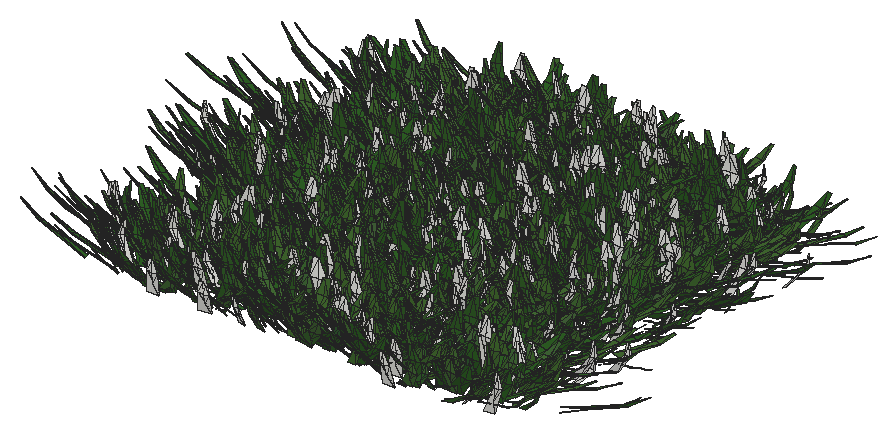
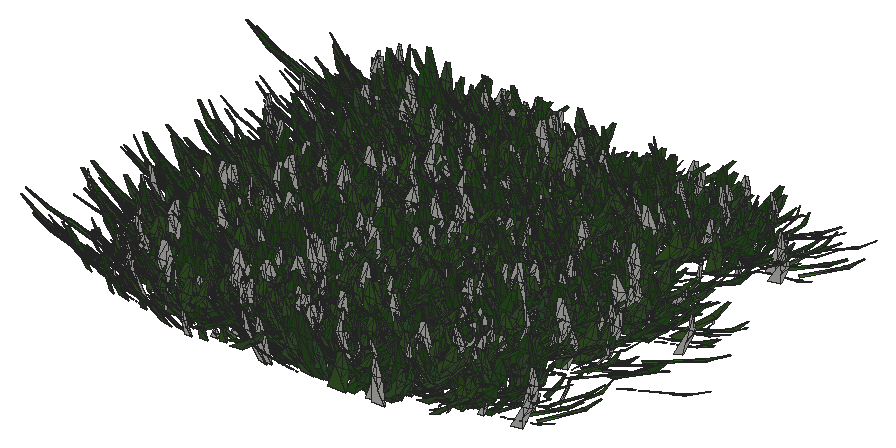
# SketchUp Ruby script. Lengths in inches.
U = 1.inch
M = Sketchup.active_model
def pt(a) = Geom::Point3d.new(a.map { |v| v * U })
def face(e, loops, mat)
  f = e.add_face(loops[0].map { |a| pt(a) })
  loops[1..].each { |l| e.add_face(l.map { |a| pt(a) }).erase! }
  f.material = f.back_material = mat if mat
  f
end
# faces: each face lists its corners as indices into pts; further lists are holes
def faces(e, pts, list, mat = nil) = list.each { |f| face(e, (f[0].is_a?(Array) ? f : [f]).map { |l| l.map { |i| pts[i] } }, mat) }
# xy, xz, yz: faces in a plane at the given z, y or x. An outline is a flat list of corners, or four numbers for a rectangle; further outlines are holes
def ring(l) = l.size == 4 ? [[l[0], l[1]], [l[2], l[1]], [l[2], l[3]], [l[0], l[3]]] : l.each_slice(2).to_a
def flat(e, list, mat, &to3) = list.each { |f| face(e, (f[0].is_a?(Array) ? f : [f]).map { |l| ring(l).map { |u, v| to3.(u, v) } }, mat) }
def xy(e, z, list, mat = nil) = flat(e, list, mat) { |x, y| [x, y, z] }
def xz(e, y, list, mat = nil) = flat(e, list, mat) { |x, z| [x, y, z] }
def yz(e, x, list, mat = nil) = flat(e, list, mat) { |y, z| [x, y, z] }
def lines(e, pts, list) = list.each { |a, b| e.add_line(pt(pts[a]), pt(pts[b])) }
# prism: a flat outline (further loops are holes) pulled along v
def prism(e, loops, v, mat = nil)
  f = face(e, loops, mat); d = Geom::Vector3d.new(v.map { |x| x * U })
  f.pushpull(f.normal.samedirection?(d) ? d.length : -d.length)
end
def box(e, o, s, mat = nil) = prism(e, [[o, [o[0] + s[0], o[1], o[2]], [o[0] + s[0], o[1] + s[1], o[2]], [o[0], o[1] + s[1], o[2]]]], [0, 0, s[2]], mat)
def at(x, y, z, deg = 0) = Geom::Transformation.translation(pt([x, y, z])) * Geom::Transformation.rotation(ORIGIN, Z_AXIS, deg.degrees)
def axes(o, x, y, z) = Geom::Transformation.new([*x, 0, *y, 0, *z, 0, *pt(o).to_a, 1])
def part(name) = M.definitions.add(name)
# library, detail: a bought-in or finely detailed component or shape, given as its bounding box
def library(name, o, s) = part(name).tap { |d| box(d.entities, o, s) }
def detail(e, o, s) = box(e.add_group.entities, o, s)
def put(e, d, t, mat = nil) = e.add_instance(d, t).tap { |i| i.material = mat if mat }
def group(e, t, mat = nil) = e.add_group.tap { |g| g.transformation = t; g.material = mat if mat }.entities
root = M.entities
M.materials.add("Material10").color = [48, 100, 38]
M.materials.add("Material3").color = [68, 110, 58]
M.materials.add("Material4").color = [48, 90, 38]
M.materials.add("Material5").color = [68, 110, 48]
M.materials.add("Material6").color = [48, 90, 48]
M.materials.add("Material7").color = [58, 110, 58]
M.materials.add("Material8").color = [58, 90, 38]
M.materials.add("Material9").color = [68, 100, 58]
c1 = part("grass00")
p = [[-0.6875,0.15,0],[-0.56,0.08,5.52],[-0.04,0.03,2.76],[0.48,-0.02,0],[0.35,-0.02,5.52],[-0.1,-0.14,5.52],
  [-0.12,0.65,8.37],[-0.42,0.65,8.37]]
faces(c1.entities,p,[[0,1,2,3],[3,2,4],[1,5,2],[5,4,2],[1,6,5],[4,5,6],[7,6,1]])
c2 = part("Group16\#1")
put(c2.entities,c1,axes([1.44,-0.61,-0.01],[0.05352,0.12609,0],[-0.10704,0.04543,0.07239],[0.06664,-0.02828,0.11628]),"Material6")
put(c2.entities,c1,axes([0.76,-0.15,-0.01],[0.04676,0.24062,0],[-0.23162,0.04501,0.06642],[0.0652,-0.01267,0.23595]),"Material3")
put(c2.entities,c1,axes([0.79,0.01,-0.01],[-0.00606,0.34651,0],[-0.34381,-0.00602,0.0432],[0.04319,0.00076,0.34386]))
put(c2.entities,c1,axes([1,0.23,-0.01],[-0.07192,0.31144,0],[-0.28722,-0.06632,0.1236],[0.12043,0.02781,0.29478]),"Material5")
put(c2.entities,c1,axes([1.66,0.77,-0.01],[-0.13828,0.29651,0],[-0.21551,-0.1005,0.22471],[0.20365,0.09498,0.23779]),"Material10")
put(c2.entities,c1,axes([0.6875,0.52,-0.01],[-0.18126,0.24051,0],[-0.22746,-0.17142,0.09788],[0.07817,0.05891,0.28481]),"Material5")
put(c2.entities,c1,axes([0.68,0.78,-0.01],[-0.215,0.18688,0],[-0.12385,-0.14248,0.21334],[0.13995,0.16101,0.18878]),"Material3")
put(c2.entities,c1,axes([0.56,1,-0.01],[-0.13756,0.07624,0],[-0.06159,-0.11112,0.0927],[0.04494,0.08108,0.12705]),"Material5")
put(c2.entities,c1,axes([0.2,0.64,-0.01],[-0.23729,0.07254,0],[-0.05711,-0.18681,0.153],[0.04473,0.14632,0.19535]),"Material10")
put(c2.entities,c1,axes([0.0625,0.72,-0.01],[-0.28874,0.02525,0],[-0.02179,-0.24916,0.14647],[0.01276,0.14591,0.25012]),"Material3")
put(c2.entities,c1,axes([-0.08,0.62,-0.01],[-0.34089,-0.04187,0],[0.03255,-0.26504,0.216],[-0.02633,0.21439,0.26703]),"Material10")
put(c2.entities,c1,axes([-0.34,0.98,-0.01],[-0.14314,-0.0493,0],[0.04397,-0.12769,0.06843],[-0.02228,0.0647,0.13505]),"Material10")
put(c2.entities,c1,axes([-0.87,1.45,-0.01],[-0.23488,-0.14114,0],[0.13761,-0.22901,0.06087],[-0.03135,0.05217,0.26717]))
put(c2.entities,c1,axes([-0.72,0.77,-0.01],[-0.14208,-0.13251,0],[0.07209,-0.0773,0.16301],[-0.11118,0.11922,0.1057]),"Material10")
put(c2.entities,c1,axes([-0.62,0.43,-0.01],[-0.14845,-0.21203,0],[0.18654,-0.13061,0.12304],[-0.10079,0.07057,0.22772]),"Material3")
put(c2.entities,c1,axes([-0.68,0.29,-0.01],[-0.13639,-0.32136,0],[0.31723,-0.13464,0.05579],[-0.05136,0.0218,0.34462]),"Material4")
put(c2.entities,c1,axes([-0.64,0.125,-0.01],[-0.0458,-0.23569,0],[0.22124,-0.043,0.08276],[-0.08124,0.01579,0.22538]),"Material7")
put(c2.entities,c1,axes([-1.6,-0.03,-0.01],[0.00576,-0.32897,0],[0.27526,0.00482,0.18018],[-0.18015,-0.00315,0.2753]),"Material5")
put(c2.entities,c1,axes([-1.36,-0.31,-0.01],[0.05718,-0.24765,0],[0.18172,0.04196,0.17267],[-0.16825,-0.03885,0.1865]),"Material10")
put(c2.entities,c1,axes([-1.54,-0.72,-0.01],[0.06537,-0.14017,0],[0.13555,0.06321,0.03939],[-0.0357,-0.01665,0.14956]))
put(c2.entities,c1,axes([-1.19,-0.9,-0.01],[0.09597,-0.12735,0],[0.11214,0.08451,0.07557],[-0.06035,-0.04548,0.14042]),"Material9")
put(c2.entities,c1,axes([-0.47,-0.54,-0.01],[0.11588,-0.10072,0],[0.0618,0.0711,0.12124],[-0.07953,-0.0915,0.0942]))
put(c2.entities,c1,axes([-0.47,-0.84,-0.01],[0.11927,-0.0661,0],[0.06603,0.11913,0.00646],[-0.00313,-0.00565,0.13621]),"Material5")
put(c2.entities,c1,axes([-0.38,-1.24,-0.01],[0.28037,-0.08571,0],[0.0618,0.20215,0.20315],[-0.05939,-0.19428,0.21139]),"Material9")
put(c2.entities,c1,axes([-0.06,-0.66,-0.01],[0.22719,-0.01987,0],[0.01247,0.14255,0.17758],[-0.01547,-0.17691,0.1431]),"Material8")
put(c2.entities,c1,axes([0.11,-0.89,-0.01],[0.14882,0.01828,0],[-0.01058,0.08611,0.12229],[0.01491,-0.12138,0.08676]),"Material6")
put(c2.entities,c1,axes([0.25,-0.72,-0.01],[0.20481,0.07053,0],[-0.06206,0.18022,0.10291],[0.03351,-0.0973,0.1906]),"Material6")
put(c2.entities,c1,axes([0.85,-1.42,-0.01],[0.16481,0.09904,0],[-0.09472,0.15762,0.05616],[0.02893,-0.04814,0.18389]),"Material5")
put(c2.entities,c1,axes([1.01,-1.09,-0.01],[0.21858,0.20385,0],[-0.17495,0.1876,0.15339],[0.10462,-0.11218,0.25652]),"Material10")
put(c2.entities,c1,axes([1.01,-0.71,-0.01],[0.08733,0.12473,0],[-0.06445,0.04512,0.13037],[0.1068,-0.07477,0.07867]),"Material6")
c3 = part("Group15\#1")
put(c3.entities,c2,at(0,0,0))
c4 = part("3darcstudiotree_grass00\#1")
put(c4.entities,c3,at(0,0,0))
put(root,c4,axes([225.51,46.77,7.6],[3.32161,0.35112,0],[-1.50903,0.89222,-0.04149],[-0.12715,0.07518,1.90578]))
put(root,c4,axes([225.43,47.55,7.6],[4.42522,0.39878,0],[-1.59159,1.10387,-0.05978],[-0.10331,0.07165,1.49495]))
put(root,c4,axes([226.83,43.55,7.6],[-3.44676,0.28749,0],[-1.23509,-0.92549,-0.01591],[-0.0303,-0.02271,1.46774]))
put(root,c4,axes([225.29,62.01,7.6],[3.38445,0.8074,0],[-3.01391,0.7896,-0.00767],[-0.03555,0.00931,1.8325]))
put(root,c4,axes([226.57,49.54,7.6],[1.69893,-0.90725,0],[3.27841,0.3837,-0.04141],[0.32735,0.03831,1.97468]))
put(root,c4,axes([225.81,75.55,7.6],[3.91819,0.15531,0],[-0.72225,1.13884,-0.02805],[-0.0304,0.04793,1.99488]))
put(root,c4,axes([227.24,69.53,7.6],[-4.474,0.54268,0],[-2.22283,-1.14534,-0.06144],[-0.11475,-0.05913,1.3618]))
put(root,c4,axes([226.4,58.8,7.6],[4.53734,-0.32224,0],[1.09679,0.96521,-0.02465],[0.03792,0.03337,1.41248]))
put(root,c4,axes([227.88,65.96,7.6],[-4.98405,0.08955,0],[-0.32681,-1.13684,-0.01837],[-0.00709,-0.02466,1.53349]))
put(root,c4,axes([226.71,68.04,7.6],[-2.12527,0.78662,0],[-4.24604,-0.71699,-0.01862],[-0.09082,-0.01534,1.88514]))
put(root,c4,axes([226.98,57.51,7.6],[-0.84491,0.92662,0],[-3.59657,-0.20496,-0.03421],[-0.27144,-0.01547,1.87625]))
put(root,c4,axes([226.67,78.54,7.6],[4.27273,0.49757,0],[-1.69118,0.90766,-0.0112],[-0.0297,0.01594,1.5714]))
put(root,c4,axes([227.35,59.97,7.6],[-2.09567,1.0755,0],[-4.66144,-0.56769,-0.00711],[-0.02652,-0.00323,1.34501]))
put(root,c4,axes([228.02,63.18,7.6],[3.76579,0.18942,0],[-0.73722,0.91603,-0.0192],[-0.02664,0.0331,1.64321]))
put(root,c4,axes([229.68,47.52,7.6],[-4.50451,-0.0411,0],[0.16437,-1.12587,-0.04384],[0.00948,-0.0649,1.66887]))
put(root,c4,axes([230.15,67.33,7.6],[1.13978,-1.18562,0],[3.93385,0.23636,-0.00397],[0.02802,0.00168,1.83602]))
put(root,c4,axes([229.77,78.18,7.6],[2.04927,-1.15149,0],[3.67293,0.40854,-0.03607],[0.18559,0.02064,1.41495]))
put(root,c4,axes([230.57,46.05,7.6],[-3.89235,0.6193,0],[-1.97046,-0.77403,-0.04609],[-0.18429,-0.07239,1.7083]))
put(root,c4,axes([230.76,71.03,7.6],[-4.69047,0.29817,0],[-0.94339,-0.92751,-0.01716],[-0.03313,-0.03258,1.87475]))
put(root,c4,axes([231.34,49.36,7.6],[-2.56498,-0.70635,0],[3.60094,-0.81726,-0.05879],[0.23789,-0.05399,1.66118]))
put(root,c4,axes([229.9,65.69,7.6],[2.78646,0.69678,0],[-2.91891,0.72956,-0.04694],[-0.21834,0.05457,1.69685]))
put(root,c4,axes([230.3,61.375,7.6],[4.00096,-0.34776,0],[1.36846,0.984,-0.02118],[0.04627,0.03327,1.73224]))
put(root,c4,axes([231.29,44.32,7.6],[-3.88364,0.22634,0],[-1.16126,-1.24533,-0.06463],[-0.06106,-0.06548,1.33032]))
put(root,c4,axes([231.57,58.36,7.6],[-0.3144,-1.12257,0],[4.53452,-0.07937,-0.04142],[0.25114,-0.0044,1.72685]))
put(root,c4,axes([229.6,69.17,7.6],[2.22373,1.05105,0],[-4.23729,0.56031,-0.01033],[-0.04653,0.00615,1.52631]))
put(root,c4,axes([230.13,63.06,7.6],[1.40015,0.90192,0],[-4.40254,0.42716,-0.04732],[-0.21206,0.02058,1.41896]))
put(root,c4,axes([232.17,79.92,7.6],[-2.10821,-0.79686,0],[3.44011,-0.56883,-0.00554],[0.0286,-0.00473,1.59445]))
put(root,c4,axes([230.7,51.86,7.6],[-2.15643,1.07136,0],[-4.45067,-0.55989,-0.00338],[-0.01774,-0.00223,1.82725]))
put(root,c4,axes([232.37,73.84,7.6],[-1.26196,-1.16235,0],[3.99848,-0.27132,-0.0298],[0.15935,-0.01081,1.43464]))
put(root,c4,axes([232.38,51.15,7.6],[-3.90512,0.37554,0],[-1.32571,-0.86161,-0.01112],[-0.02945,-0.01914,1.70172]))
put(root,c4,axes([231.08,59.87,7.6],[3.89687,0.53963,0],[-2.2724,1.02562,-0.02111],[-0.06659,0.03005,1.90804]))
put(root,c4,axes([231.65,56.78,7.6],[4.64847,0.14796,0],[-0.47459,0.93187,-0.04636],[-0.04617,0.09067,1.85211]))
put(root,c4,axes([232.62,75.15,7.6],[-3.09239,0.5801,0],[-2.93834,-0.97897,-0.02868],[-0.07819,-0.02605,1.39]))
put(root,c4,axes([233.83,55.11,7.6],[-4.25986,-0.54269,0],[2.31668,-1.13655,-0.02171],[0.04865,-0.02387,1.57387]))
put(root,c4,axes([233.84,64.58,7.6],[-2.77535,-0.81036,0],[3.4317,-0.73456,-0.03189],[0.13148,-0.02814,1.53238]))
put(root,c4,axes([232.95,81.42,7.6],[3.79578,-0.24018,0],[1.14982,1.13575,-0.03471],[0.05624,0.05555,1.93398]))
put(root,c4,axes([233.49,77.125,7.6],[-2.12934,0.97427,0],[-4.32415,-0.59067,-0.04785],[-0.24231,-0.0331,1.77706]))
put(root,c4,axes([233.25,71.55,7.6],[4.30806,0.2682,0],[-1.01562,1.01959,-0.04825],[-0.06479,0.06504,1.45973]))
put(root,c4,axes([233.85,53.98,7.6],[3.59575,0.08404,0],[-0.42601,1.13924,-0.04931],[-0.02468,0.066,1.538]))
put(root,c4,axes([236.91,55.09,7.6],[-3.88808,0.63083,0],[-2.21629,-0.85375,-0.02727],[-0.08235,-0.03172,1.41127]))
put(root,c4,axes([237.78,75.52,7.6],[-1.09356,-0.98806,0],[3.47695,-0.24051,-0.0133],[0.08295,-0.00574,1.45899]))
put(root,c4,axes([236.04,71.8125,7.6],[3.11671,0.55561,0],[-2.5205,0.88368,-0.03635],[-0.10975,0.03848,1.41103]))
put(root,c4,axes([236.42,58.55,7.6],[1.23042,1.06401,0],[-3.79842,0.27453,-0.04889],[-0.27893,0.02016,1.46761]))
put(root,c4,axes([237.69,82.22,7.6],[1.50651,-0.83711,0],[4.29011,0.48255,-0.04402],[0.24827,0.02793,1.81837]))
put(root,c4,axes([238.48,67.36,7.6],[-4.37435,-0.52642,0],[1.61836,-0.8405,-0.01121],[0.03956,-0.02054,1.89718]))
put(root,c4,axes([236.35,70.68,7.6],[4.06113,0.54294,0],[-1.83498,0.85783,-0.00407],[-0.01255,0.00587,1.59208]))
put(root,c4,axes([238.12,48.05,7.6],[1.79956,-0.79311,0],[4.48938,0.63665,-0.03953],[0.18894,0.02679,1.77239]))
put(root,c4,axes([236.78,46.68,7.6],[0.4509,1.27151,0],[-4.34293,0.09625,-0.0152],[-0.08927,0.00198,1.60635]))
put(root,c4,axes([239.13,50.46,7.6],[0.25819,-1.20405,0],[5.15523,0.06909,-0.00697],[0.04087,0.00055,1.89407]))
put(root,c4,axes([238.91,53.71,7.6],[-3.83272,-0.39572,0],[1.58422,-0.959,-0.04671],[0.12739,-0.07712,1.85324]))
put(root,c4,axes([239,80.97,7.6],[-3.58122,-0.18152,0],[0.97164,-1.19807,-0.02938],[0.02523,-0.03112,1.3208]))
put(root,c4,axes([237.9,49.125,7.6],[1.00148,1.21567,0],[-4.0422,0.20812,-0.03105],[-0.22157,0.01141,1.87912]))
put(root,c4,axes([237.5625,76.51,7.6],[1.9958,1.15638,0],[-4.53864,0.48958,-0.02206],[-0.10786,0.01163,1.64521]))
put(root,c4,axes([238.1875,52.41,7.6],[1.40221,1.20778,0],[-3.61732,0.26248,-0.03743],[-0.21438,0.01556,1.40382]))
put(root,c4,axes([239.33,79.27,7.6],[3.20601,-0.72944,0],[2.8275,0.7767,-0.00947],[0.03301,0.00907,1.36019]))
put(root,c4,axes([238.73,59.83,7.6],[2.6445,0.64267,0],[-3.36196,0.86462,-0.04673],[-0.15716,0.04042,1.45453]))
put(root,c4,axes([239.22,61.22,7.6],[4.6939,-0.33478,0],[1.42081,1.24507,-0.04256],[0.05609,0.04915,1.55488]))
put(root,c4,axes([239.58,62.5,7.6],[0.70081,1.13515,0],[-3.837,0.14805,-0.04631],[-0.31213,0.01204,1.65491]))
put(root,c4,axes([239.43,73.13,7.6],[0.79643,0.97824,0],[-4.073,0.20725,-0.02796],[-0.20539,0.01045,1.94708]))
put(root,c4,axes([240.1,57.1,7.6],[4.47521,-0.51509,0],[1.59075,0.86381,-0.00355],[0.00999,0.00542,1.60125]))
put(root,c4,axes([239.85,65.81,7.6],[3.61508,0.31151,0],[-1.17398,0.85151,-0.01199],[-0.02287,0.01659,1.31812]))
put(root,c4,axes([240.07,64.01,7.6],[1.15853,0.90177,0],[-3.74188,0.30046,-0.04361],[-0.27208,0.02185,1.60948]))
put(root,c4,axes([239.71,69.57,7.6],[4.73679,0.47209,0],[-1.3835,0.8676,-0.02018],[-0.04428,0.02777,1.38364]))
put(root,c4,axes([239.87,78.46,7.6],[3.02988,0.65339,0],[-2.92725,0.84838,-0.02494],[-0.09513,0.02757,1.63549]))
put(root,c4,axes([241.86,55.56,7.6],[-0.26338,-0.96396,0],[4.36475,-0.07454,-0.04502],[0.21373,-0.00365,1.30109]))
put(root,c4,axes([239.98,44.41,7.6],[3.70502,0.87773,0],[-2.99978,0.79141,-0.00751],[-0.03439,0.00907,1.8142]))
put(root,c4,axes([243,48.25,7.6],[1.10203,-1.11719,0],[4.19734,0.25877,-0.00763],[0.05016,0.00309,1.82848]))
put(root,c4,axes([242.39,81.72,7.6],[3.66199,-0.54584,0],[2.20621,0.92507,-0.01626],[0.05583,0.02341,1.80561]))
put(root,c4,axes([243.65,51.96,7.6],[-2.73315,-0.59238,0],[2.36909,-0.68316,-0.00893],[0.05138,-0.01482,1.98619]))
put(root,c4,axes([243.11,76.34,7.6],[2.15048,-1.04444,0],[4.49757,0.57877,-0.06088],[0.28493,0.03667,1.6642]))
put(root,c4,axes([243.65,71.16,7.6],[1.29191,-1.13081,0],[3.98569,0.2846,-0.01145],[0.06058,0.00433,1.42532]))
put(root,c4,axes([243.82,79.71,7.6],[-3.75042,-0.0193,0],[0.10511,-1.27668,-0.05231],[0.00643,-0.07814,1.90792]))
put(root,c4,axes([243.6,61.55,7.6],[2.35649,-0.70912,0],[3.7753,0.78411,-0.00974],[0.03955,0.00821,1.619]))
put(root,c4,axes([244,53.53,7.6],[-3.90716,-0.09419,0],[0.46436,-1.20386,-0.0118],[0.00503,-0.01303,1.34216]))
put(root,c4,axes([243.28,56.68,7.6],[4.63049,-0.46903,0],[1.7734,1.09423,-0.01357],[0.03424,0.02113,1.98263]))
put(root,c4,axes([242.92,78.37,7.6],[4.58241,0.19186,0],[-0.7983,1.1917,-0.00046],[-0.00036,0.00053,1.40239]))
put(root,c4,axes([243.87,64.57,7.6],[-1.84062,1.15684,0],[-3.44401,-0.34248,-0.04072],[-0.25086,-0.02495,1.53595]))
put(root,c4,axes([244.81,69.57,7.6],[-3.43993,-0.35088,0],[1.66399,-1.0196,-0.03312],[0.08822,-0.05406,1.94116]))
put(root,c4,axes([243.27,44.31,7.6],[3.69288,0.11707,0],[-0.52356,1.03223,-0.01144],[-0.00941,0.01856,1.7012]))
put(root,c4,axes([243.84,75.5,7.6],[4.06672,-0.35788,0],[1.7117,1.21566,-0.03514],[0.05649,0.04012,1.55988]))
put(root,c4,axes([243.59,49.68,7.6],[3.74539,0.69391,0],[-2.4561,0.82855,-0.03152],[-0.10739,0.03623,1.47514]))
put(root,c4,axes([245.88,45.98,7.6],[-1.01831,-1.20571,0],[4.14332,-0.21871,-0.00703],[0.03921,-0.00207,1.50812]))
put(root,c4,axes([244.35,57.91,7.6],[4.09573,-0.25172,0],[0.94943,0.96549,-0.02888],[0.04811,0.04892,1.73467]))
put(root,c4,axes([246.11,51.23,7.6],[-2.36855,-0.74824,0],[3.41575,-0.67578,-0.00813],[0.03094,-0.00612,1.32168]))
put(root,c4,axes([244.68,67.86,7.6],[-0.73359,1.07978,0],[-4.59667,-0.19518,-0.06003],[-0.37487,-0.01592,1.84592]))
put(root,c4,axes([246.21,73.1,7.6],[-2.50204,-0.67667,0],[3.03986,-0.70251,-0.01026],[0.05042,-0.01165,1.73127]))
put(root,c4,axes([244.36,62.96,7.6],[2.78719,0.78007,0],[-2.78295,0.62147,-0.01423],[-0.0832,0.01858,1.82816]))
put(root,c4,axes([246.11,71.83,7.6],[1.6891,-0.96656,0],[4.41238,0.48192,-0.02716],[0.12133,0.01325,1.46706]))
put(root,c4,axes([244.58,65.76,7.6],[1.88303,0.87084,0],[-3.91676,0.52933,-0.00296],[-0.01453,0.00196,1.55057]))
put(root,c4,axes([245.47,60.51,7.6],[-2.57647,0.98803,0],[-3.47817,-0.56688,-0.00573],[-0.03032,-0.00494,1.63969]))
put(root,c4,axes([247.76,60.3,7.6],[-3.28034,-0.7048,0],[2.67551,-0.77829,-0.00129],[0.00481,-0.0014,1.46122]))
put(root,c4,axes([248.16,45.23,7.6],[-4.50482,0.23028,0],[-0.80598,-0.98543,-0.0347],[-0.04459,-0.05452,1.61275]))
put(root,c4,axes([248.63,82.31,7.6],[-2.24979,-0.88649,0],[3.27379,-0.51928,-0.00968],[0.0585,-0.00928,1.73508]))
put(root,c4,axes([248.42,65.08,7.6],[-2.16564,-0.83911,0],[3.14801,-0.50779,-0.04434],[0.21001,-0.03388,1.31982]))
put(root,c4,axes([248.8,79.33,7.6],[-0.67756,-0.92885,0],[4.95794,-0.22604,-0.01194],[0.05933,-0.0027,1.59034]))
put(root,c4,axes([249.54,55.35,7.6],[-1.3799,-0.92069,0],[4.85694,-0.45496,-0.00645],[0.02452,-0.0023,1.31612]))
put(root,c4,axes([248.75,72.54,7.6],[-3.11177,0.67846,0],[-2.86968,-0.82262,-0.0546],[-0.24326,-0.06973,1.84968]))
put(root,c4,axes([247.79,49.89,7.6],[0.29202,1.19913,0],[-4.14046,0.06302,-0.02381],[-0.16303,0.00248,1.77807]))
put(root,c4,axes([249.15,56.59,7.6],[0.24548,-1.00327,0],[4.53075,0.06929,-0.05271],[0.25543,0.00391,1.37729]))
put(root,c4,axes([248.9,45.78,7.6],[2.19726,-0.80915,0],[3.02534,0.51346,-0.03969],[0.20361,0.03456,1.41714]))
put(root,c4,axes([248.93,73.1,7.6],[-3.397,0.74366,0],[-2.61152,-0.74558,-0.00238],[-0.01206,-0.00344,1.90825]))
put(root,c4,axes([249.89,54.35,7.6],[-3.12263,-0.80969,0],[2.7475,-0.66225,-0.03577],[0.16124,-0.03886,1.49339]))
put(root,c4,axes([248.54,52.41,7.6],[1.11929,0.91122,0],[-4.49159,0.34483,-0.03259],[-0.18787,0.01442,1.77089]))
put(root,c4,axes([248.65,77.6875,7.6],[0.31588,1.13425,0],[-4.04106,0.07034,-0.01352],[-0.07984,0.00139,1.49862]))
put(root,c4,axes([248.55,62.03,7.6],[3.21264,0.8518,0],[-2.81244,0.66296,-0.02839],[-0.16121,0.038,1.88589]))
put(root,c4,axes([250.64,58.97,7.6],[-0.18941,-0.91577,0],[4.95051,-0.06399,-0.00424],[0.02167,-0.00028,1.58408]))
put(root,c4,axes([250.9375,80.72,7.6],[-4.97788,-0.34272,0],[1.27823,-1.16037,-0.00177],[0.00271,-0.00246,1.73275]))
put(root,c4,axes([249.7,70.8,7.6],[3.21803,-0.64979,0],[2.61533,0.80951,-0.03491],[0.156,0.04829,1.84986]))
put(root,c4,axes([249.89,75.45,7.6],[-2.15492,0.7494,0],[-3.61151,-0.64906,-0.0015],[-0.00592,-0.00106,1.35234]))
put(root,c4,axes([251.88,50.87,7.6],[-4.78225,-0.48138,0],[1.79554,-1.11486,-0.01703],[0.03477,-0.02159,1.64249]))
put(root,c4,axes([251.33,43.69,7.6],[-3.37934,0.52143,0],[-1.92704,-0.78055,-0.03387],[-0.1051,-0.04257,1.3548]))
put(root,c4,axes([251.89,62.88,7.6],[-4.43307,0.16391,0],[-0.66186,-1.11881,-0.04443],[-0.04202,-0.07104,1.82802]))
put(root,c4,axes([250.29,47.77,7.6],[3.59313,0.68873,0],[-2.26385,0.73816,-0.03117],[-0.10632,0.03467,1.30357]))
put(root,c4,axes([250.49,76.74,7.6],[-0.883,1.08324,0],[-4.56364,-0.2325,-0.00834],[-0.04858,-0.00247,1.72954]))
put(root,c4,axes([251.79,66.42,7.6],[3.26656,-0.94634,0],[3.22899,0.69661,-0.04774],[0.259,0.05588,1.91023]))
put(root,c4,axes([250.96,67.23,7.6],[1.182,1.03878,0],[-4.83466,0.34383,-0.01266],[-0.06647,0.00473,1.71446]))
put(root,c4,axes([251.83,69.2,7.6],[3.68181,-0.04873,0],[0.19766,0.93331,-0.02933],[0.01311,0.06192,1.97542]))
put(root,c4,axes([254.1,58.93,7.6],[-3.47365,-0.63097,0],[2.73432,-0.94081,-0.03763],[0.14803,-0.05093,1.94544]))
put(root,c4,axes([254.46,52.54,7.6],[-3.67495,-0.82991,0],[3.18036,-0.88019,-0.0585],[0.25242,-0.06986,1.90866]))
put(root,c4,axes([254.3125,64.5,7.6],[1.84359,-0.98578,0],[4.27522,0.49972,-0.01397],[0.07469,0.00873,1.74087]))
put(root,c4,axes([254.94,70.93,7.6],[-2.66867,-0.63345,0],[3.02701,-0.79703,-0.01822],[0.08532,-0.02247,1.86907]))
put(root,c4,axes([253.82,57.49,7.6],[-1.38022,0.90937,0],[-3.69449,-0.35046,-0.03389],[-0.21225,-0.02013,1.65454]))
put(root,c4,axes([255.12,45.15,7.6],[-3.71907,-0.26708,0],[1.32824,-1.15597,-0.05258],[0.08896,-0.07742,1.84274]))
put(root,c4,axes([255.65,71.7,7.6],[-3.44494,-0.92514,0],[2.808,-0.65351,-0.04944],[0.24269,-0.05648,1.60821]))
put(root,c4,axes([254.68,81.2,7.6],[-1.24544,1.08485,0],[-3.56774,-0.25599,-0.04255],[-0.31037,-0.02227,1.76068]))
put(root,c4,axes([255.59,50.33,7.6],[-0.08294,-1.02259,0],[4.8002,-0.02433,-0.05384],[0.23738,-0.0012,1.32332]))
put(root,c4,axes([255.5625,53.79,7.6],[-3.9311,-0.05315,0],[0.20584,-0.95146,-0.00522],[0.00166,-0.00767,1.40302]))
put(root,c4,axes([255.64,61.9,7.6],[-4.14008,0.40448,0],[-1.31245,-0.8396,-0.02866],[-0.08715,-0.05575,1.88291]))
put(root,c4,axes([256.48,55.87,7.6],[-3.68165,-0.61094,0],[2.8571,-1.07609,-0.03911],[0.09635,-0.03629,1.43856]))
put(root,c4,axes([255.875,49.02,7.6],[-0.00357,-0.95329,0],[3.72251,-0.00087,-0.0371],[0.29437,-0.00007,1.84609]))
put(root,c4,axes([256.73,62.86,7.6],[-3.07811,-0.52655,0],[2.38746,-0.87229,-0.01797],[0.0526,-0.01922,1.36964]))
put(root,c4,axes([255.72,48.33,7.6],[3.95966,-0.70893,0],[2.92387,1.02069,-0.04389],[0.15667,0.05469,1.92393]))
put(root,c4,axes([257.36,73.51,7.6],[-2.20402,-1.1259,0],[4.50927,-0.5517,-0.06506],[0.31838,-0.03895,1.70958]))
put(root,c4,axes([257.23,68.5625,7.6],[1.30701,-0.93257,0],[4.74609,0.41573,-0.02001],[0.10664,0.00934,1.77455]))
put(root,c4,axes([256.89,74.91,7.6],[2.24839,-0.79603,0],[3.33272,0.58833,-0.00946],[0.04896,0.00864,1.61646]))
put(root,c4,axes([256.07,79.5,7.6],[-1.06084,1.03088,0],[-4.97495,-0.31997,-0.03008],[-0.16035,-0.01031,1.76703]))
put(root,c4,axes([255.83,66.24,7.6],[3.29499,0.88006,0],[-3.34052,0.78169,-0.05678],[-0.19382,0.04535,1.337]))
put(root,c4,axes([256.87,46.76,7.6],[4.12637,-0.29278,0],[1.25845,1.1085,-0.03157],[0.05307,0.04674,1.77323]))
put(root,c4,axes([256.59,78.41,7.6],[3.81538,0.13844,0],[-0.69714,1.20077,-0.0224],[-0.01503,0.02589,1.41716]))
put(root,c4,axes([257.19,76.31,7.6],[3.87873,-0.1816,0],[0.87965,1.17427,-0.05648],[0.04872,0.06503,1.39957]))
put(root,c4,axes([257.2,59.82,7.6],[2.2908,0.71526,0],[-3.14647,0.62983,-0.01526],[-0.09231,0.01848,1.9517]))
put(root,c4,axes([257.45,67.57,7.6],[1.88546,0.82083,0],[-4.0871,0.58676,-0.0451],[-0.25686,0.03688,1.93445]))
